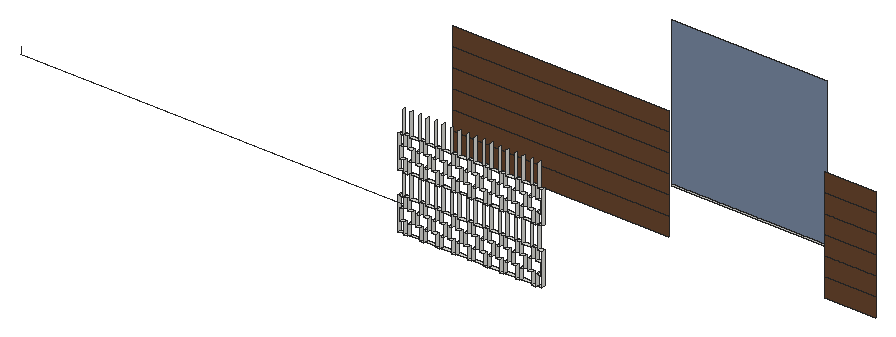
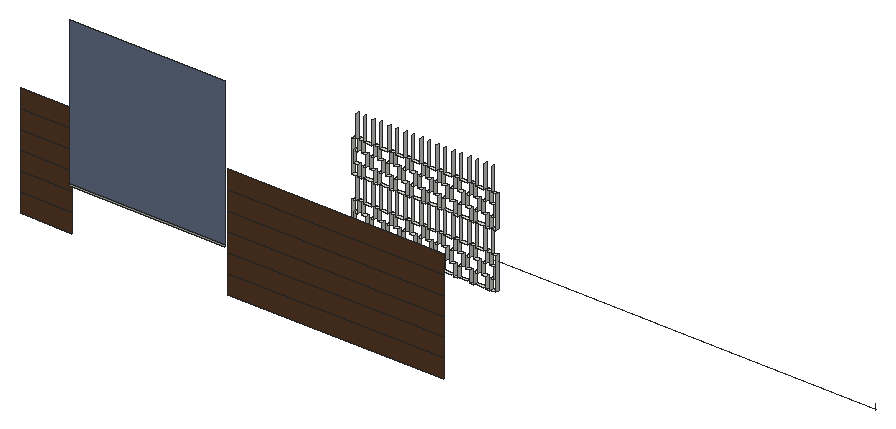
# SketchUp Ruby script. Lengths in inches.
U = 1.inch
M = Sketchup.active_model
def pt(a) = Geom::Point3d.new(a.map { |v| v * U })
def face(e, loops, mat)
  f = e.add_face(loops[0].map { |a| pt(a) })
  loops[1..].each { |l| e.add_face(l.map { |a| pt(a) }).erase! }
  f.material = f.back_material = mat if mat
  f
end
# faces: each face lists its corners as indices into pts; further lists are holes
def faces(e, pts, list, mat = nil) = list.each { |f| face(e, (f[0].is_a?(Array) ? f : [f]).map { |l| l.map { |i| pts[i] } }, mat) }
# xy, xz, yz: faces in a plane at the given z, y or x. An outline is a flat list of corners, or four numbers for a rectangle; further outlines are holes
def ring(l) = l.size == 4 ? [[l[0], l[1]], [l[2], l[1]], [l[2], l[3]], [l[0], l[3]]] : l.each_slice(2).to_a
def flat(e, list, mat, &to3) = list.each { |f| face(e, (f[0].is_a?(Array) ? f : [f]).map { |l| ring(l).map { |u, v| to3.(u, v) } }, mat) }
def xy(e, z, list, mat = nil) = flat(e, list, mat) { |x, y| [x, y, z] }
def xz(e, y, list, mat = nil) = flat(e, list, mat) { |x, z| [x, y, z] }
def yz(e, x, list, mat = nil) = flat(e, list, mat) { |y, z| [x, y, z] }
def lines(e, pts, list) = list.each { |a, b| e.add_line(pt(pts[a]), pt(pts[b])) }
# prism: a flat outline (further loops are holes) pulled along v
def prism(e, loops, v, mat = nil)
  f = face(e, loops, mat); d = Geom::Vector3d.new(v.map { |x| x * U })
  f.pushpull(f.normal.samedirection?(d) ? d.length : -d.length)
end
def box(e, o, s, mat = nil) = prism(e, [[o, [o[0] + s[0], o[1], o[2]], [o[0] + s[0], o[1] + s[1], o[2]], [o[0], o[1] + s[1], o[2]]]], [0, 0, s[2]], mat)
def at(x, y, z, deg = 0) = Geom::Transformation.translation(pt([x, y, z])) * Geom::Transformation.rotation(ORIGIN, Z_AXIS, deg.degrees)
def axes(o, x, y, z) = Geom::Transformation.new([*x, 0, *y, 0, *z, 0, *pt(o).to_a, 1])
def part(name) = M.definitions.add(name)
# library, detail: a bought-in or finely detailed component or shape, given as its bounding box
def library(name, o, s) = part(name).tap { |d| box(d.entities, o, s) }
def detail(e, o, s) = box(e.add_group.entities, o, s)
def put(e, d, t, mat = nil) = e.add_instance(d, t).tap { |i| i.material = mat if mat }
def group(e, t, mat = nil) = e.add_group.tap { |g| g.transformation = t; g.material = mat if mat }.entities
root = M.entities
M.materials.add("Glass_Mirror_01").color = [119, 135, 160]
M.materials.add("Wood_Veneer_15_1K").color = [103, 69, 45]
xy(root,322.72,[[283.14,137.21,284.89,138.74],[290.55,137.21,292.3,138.74],[297.96,137.21,299.71,138.74],[305.37,137.21,307.12,138.74],[312.78,137.21,314.53,138.74],
  [320.1875,137.21,321.94,138.74],[327.6,137.21,329.35,138.74],[335.01,137.21,336.76,138.74],[342.42,137.21,344.17,138.74]])
xy(root,323.12,[[280.31,137.21,282.27,138.74],[285.76,137.21,289.68,138.74],[293.17,137.21,297.09,138.74],[300.58,137.21,304.5,138.74],[307.99,137.21,311.91,138.74],
  [315.4,137.21,319.32,138.74],[322.81,137.21,326.73,138.74],[330.22,137.21,334.14,138.74],[337.63,137.21,341.55,138.74],[345.04,137.21,347,138.74]])
xy(root,327.99,[[281.18,137.21,283.14,138.74],[284.89,137.21,286.85,138.74],[288.59,137.21,290.55,138.74],[292.3,137.21,294.26,138.74],[296,137.21,297.96,138.74],
  [299.71,137.21,301.67,138.74],[303.41,137.21,305.37,138.74],[307.12,137.21,309.08,138.74],[310.82,137.21,312.78,138.74],[314.53,137.21,316.49,138.74],
  [318.23,137.21,320.1875,138.74],[321.94,137.21,323.9,138.74],[325.64,137.21,327.6,138.74],[329.35,137.21,331.31,138.74],[333.05,137.21,335.01,138.74],
  [336.76,137.21,338.72,138.74],[340.46,137.21,342.42,138.74],[344.17,137.21,346.13,138.74]])
xy(root,333.35,[[281.18,137.21,283.14,138.74],[284.89,137.21,286.85,138.74],[288.59,137.21,290.55,138.74],[292.3,137.21,294.26,138.74],[296,137.21,297.96,138.74],
  [299.71,137.21,301.67,138.74],[303.41,137.21,305.37,138.74],[307.12,137.21,309.08,138.74],[310.82,137.21,312.78,138.74],[314.53,137.21,316.49,138.74],
  [318.23,137.21,320.1875,138.74],[321.94,137.21,323.9,138.74],[325.64,137.21,327.6,138.74],[329.35,137.21,331.31,138.74],[333.05,137.21,335.01,138.74],
  [336.76,137.21,338.72,138.74],[340.46,137.21,342.42,138.74],[344.17,137.21,346.13,138.74]])
xy(root,338.22,[[280.31,137.21,282.27,138.74],[285.76,137.21,289.68,138.74],[293.17,137.21,297.09,138.74],[300.58,137.21,304.5,138.74],[307.99,137.21,311.91,138.74],
  [315.4,137.21,319.32,138.74],[322.81,137.21,326.73,138.74],[330.22,137.21,334.14,138.74],[337.63,137.21,341.55,138.74],[345.04,137.21,347,138.74]])
xy(root,338.62,[[283.14,137.21,284.89,138.74],[290.55,137.21,292.3,138.74],[297.96,137.21,299.71,138.74],[305.37,137.21,307.12,138.74],[312.78,137.21,314.53,138.74],
  [320.1875,137.21,321.94,138.74],[327.6,137.21,329.35,138.74],[335.01,137.21,336.76,138.74],[342.42,137.21,344.17,138.74]])
xy(root,348.35,[[283.14,137.21,284.89,138.74],[290.55,137.21,292.3,138.74],[297.96,137.21,299.71,138.74],[305.37,137.21,307.12,138.74],[312.78,137.21,314.53,138.74],
  [320.1875,137.21,321.94,138.74],[327.6,137.21,329.35,138.74],[335.01,137.21,336.76,138.74],[342.42,137.21,344.17,138.74]])
xy(root,348.75,[[280.31,137.21,282.27,138.74],[285.76,137.21,289.68,138.74],[293.17,137.21,297.09,138.74],[300.58,137.21,304.5,138.74],[307.99,137.21,311.91,138.74],
  [315.4,137.21,319.32,138.74],[322.81,137.21,326.73,138.74],[330.22,137.21,334.14,138.74],[337.63,137.21,341.55,138.74],[345.04,137.21,347,138.74]])
xy(root,353.62,[[281.18,137.21,283.14,138.74],[284.89,137.21,286.85,138.74],[288.59,137.21,290.55,138.74],[292.3,137.21,294.26,138.74],[296,137.21,297.96,138.74],
  [299.71,137.21,301.67,138.74],[303.41,137.21,305.37,138.74],[307.12,137.21,309.08,138.74],[310.82,137.21,312.78,138.74],[314.53,137.21,316.49,138.74],
  [318.23,137.21,320.1875,138.74],[321.94,137.21,323.9,138.74],[325.64,137.21,327.6,138.74],[329.35,137.21,331.31,138.74],[333.05,137.21,335.01,138.74],
  [336.76,137.21,338.72,138.74],[340.46,137.21,342.42,138.74],[344.17,137.21,346.13,138.74]])
xy(root,358.98,[[281.18,137.21,283.14,138.74],[284.89,137.21,286.85,138.74],[288.59,137.21,290.55,138.74],[292.3,137.21,294.26,138.74],[296,137.21,297.96,138.74],
  [299.71,137.21,301.67,138.74],[303.41,137.21,305.37,138.74],[307.12,137.21,309.08,138.74],[310.82,137.21,312.78,138.74],[314.53,137.21,316.49,138.74],
  [318.23,137.21,320.1875,138.74],[321.94,137.21,323.9,138.74],[325.64,137.21,327.6,138.74],[329.35,137.21,331.31,138.74],[333.05,137.21,335.01,138.74],
  [336.76,137.21,338.72,138.74],[340.46,137.21,342.42,138.74],[344.17,137.21,346.13,138.74]])
xy(root,363.84,[[280.31,137.21,282.27,138.74],[285.76,137.21,289.68,138.74],[293.17,137.21,297.09,138.74],[300.58,137.21,304.5,138.74],[307.99,137.21,311.91,138.74],
  [315.4,137.21,319.32,138.74],[322.81,137.21,326.73,138.74],[330.22,137.21,334.14,138.74],[337.63,137.21,341.55,138.74],[345.04,137.21,347,138.74]])
xy(root,364.24,[[283.14,137.21,284.89,138.74],[290.55,137.21,292.3,138.74],[297.96,137.21,299.71,138.74],[305.37,137.21,307.12,138.74],[312.78,137.21,314.53,138.74],
  [320.1875,137.21,321.94,138.74],[327.6,137.21,329.35,138.74],[335.01,137.21,336.76,138.74],[342.42,137.21,344.17,138.74]])
xz(root,198,[[256.9,321.28,357,329.96],[429,321.28,453,329.96],[256.9,329.96,357,338.64],[429,329.96,453,338.64],[256.9,338.64,357,347.32],
  [429,338.64,453,347.32],[256.9,347.32,357,356],[429,347.32,453,356],[256.9,356,357,364.68],[429,356,453,364.68],
  [256.9,364.68,357,373.36],[429,364.68,453,373.36]],"Wood_Veneer_15_1K")
xz(root,199.5,[[357,341.52,429,342.52]])
xz(root,199.5,[[357,342.52,429,410.35]],"Glass_Mirror_01")
yz(root,280.31,[[137.21,323.12,138.74,338.22],[137.21,348.75,138.74,363.84]])
yz(root,281.18,[[137.21,327.99,138.74,333.35],[137.21,353.62,138.74,358.98]])
yz(root,282.27,[[137.21,338.22,138.74,348.75],[137.21,363.84,138.74,374.38]])
yz(root,283.14,[[137.21,322.72,138.74,327.99],[137.21,333.35,138.74,338.62],[137.21,348.35,138.74,353.62],[137.21,358.98,138.74,364.24]])
yz(root,284.89,[[137.21,322.72,138.74,327.99],[137.21,333.35,138.74,338.62],[137.21,348.35,138.74,353.62],[137.21,358.98,138.74,364.24]])
yz(root,285.76,[[137.21,338.22,138.74,348.75],[137.21,363.84,138.74,374.38]])
yz(root,286.85,[[137.21,327.99,138.74,333.35],[137.21,353.62,138.74,358.98]])
yz(root,288.59,[[137.21,327.99,138.74,333.35],[137.21,353.62,138.74,358.98]])
yz(root,289.68,[[137.21,338.22,138.74,348.75],[137.21,363.84,138.74,374.38]])
yz(root,290.55,[[137.21,322.72,138.74,327.99],[137.21,333.35,138.74,338.62],[137.21,348.35,138.74,353.62],[137.21,358.98,138.74,364.24]])
yz(root,292.3,[[137.21,322.72,138.74,327.99],[137.21,333.35,138.74,338.62],[137.21,348.35,138.74,353.62],[137.21,358.98,138.74,364.24]])
yz(root,293.17,[[137.21,338.22,138.74,348.75],[137.21,363.84,138.74,374.38]])
yz(root,294.26,[[137.21,327.99,138.74,333.35],[137.21,353.62,138.74,358.98]])
yz(root,296,[[137.21,327.99,138.74,333.35],[137.21,353.62,138.74,358.98]])
yz(root,297.09,[[137.21,338.22,138.74,348.75],[137.21,363.84,138.74,374.38]])
yz(root,297.96,[[137.21,322.72,138.74,327.99],[137.21,333.35,138.74,338.62],[137.21,348.35,138.74,353.62],[137.21,358.98,138.74,364.24]])
yz(root,299.71,[[137.21,322.72,138.74,327.99],[137.21,333.35,138.74,338.62],[137.21,348.35,138.74,353.62],[137.21,358.98,138.74,364.24]])
yz(root,300.58,[[137.21,338.22,138.74,348.75],[137.21,363.84,138.74,374.38]])
yz(root,301.67,[[137.21,327.99,138.74,333.35],[137.21,353.62,138.74,358.98]])
yz(root,303.41,[[137.21,327.99,138.74,333.35],[137.21,353.62,138.74,358.98]])
yz(root,304.5,[[137.21,338.22,138.74,348.75],[137.21,363.84,138.74,374.38]])
yz(root,305.37,[[137.21,322.72,138.74,327.99],[137.21,333.35,138.74,338.62],[137.21,348.35,138.74,353.62],[137.21,358.98,138.74,364.24]])
yz(root,307.12,[[137.21,322.72,138.74,327.99],[137.21,333.35,138.74,338.62],[137.21,348.35,138.74,353.62],[137.21,358.98,138.74,364.24]])
yz(root,307.99,[[137.21,338.22,138.74,348.75],[137.21,363.84,138.74,374.38]])
yz(root,309.08,[[137.21,327.99,138.74,333.35],[137.21,353.62,138.74,358.98]])
yz(root,310.82,[[137.21,327.99,138.74,333.35],[137.21,353.62,138.74,358.98]])
yz(root,311.91,[[137.21,338.22,138.74,348.75],[137.21,363.84,138.74,374.38]])
yz(root,312.78,[[137.21,322.72,138.74,327.99],[137.21,333.35,138.74,338.62],[137.21,348.35,138.74,353.62],[137.21,358.98,138.74,364.24]])
yz(root,314.53,[[137.21,322.72,138.74,327.99],[137.21,333.35,138.74,338.62],[137.21,348.35,138.74,353.62],[137.21,358.98,138.74,364.24]])
yz(root,315.4,[[137.21,338.22,138.74,348.75],[137.21,363.84,138.74,374.38]])
yz(root,316.49,[[137.21,327.99,138.74,333.35],[137.21,353.62,138.74,358.98]])
yz(root,318.23,[[137.21,327.99,138.74,333.35],[137.21,353.62,138.74,358.98]])
yz(root,319.32,[[137.21,338.22,138.74,348.75],[137.21,363.84,138.74,374.38]])
yz(root,320.1875,[[137.21,322.72,138.74,327.99],[137.21,333.35,138.74,338.62],[137.21,348.35,138.74,353.62],[137.21,358.98,138.74,364.24]])
yz(root,321.94,[[137.21,322.72,138.74,327.99],[137.21,333.35,138.74,338.62],[137.21,348.35,138.74,353.62],[137.21,358.98,138.74,364.24]])
yz(root,322.81,[[137.21,338.22,138.74,348.75],[137.21,363.84,138.74,374.38]])
yz(root,323.9,[[137.21,327.99,138.74,333.35],[137.21,353.62,138.74,358.98]])
yz(root,325.64,[[137.21,327.99,138.74,333.35],[137.21,353.62,138.74,358.98]])
yz(root,326.73,[[137.21,338.22,138.74,348.75],[137.21,363.84,138.74,374.38]])
yz(root,327.6,[[137.21,322.72,138.74,327.99],[137.21,333.35,138.74,338.62],[137.21,348.35,138.74,353.62],[137.21,358.98,138.74,364.24]])
yz(root,329.35,[[137.21,322.72,138.74,327.99],[137.21,333.35,138.74,338.62],[137.21,348.35,138.74,353.62],[137.21,358.98,138.74,364.24]])
yz(root,330.22,[[137.21,338.22,138.74,348.75],[137.21,363.84,138.74,374.38]])
yz(root,331.31,[[137.21,327.99,138.74,333.35],[137.21,353.62,138.74,358.98]])
yz(root,333.05,[[137.21,327.99,138.74,333.35],[137.21,353.62,138.74,358.98]])
yz(root,334.14,[[137.21,338.22,138.74,348.75],[137.21,363.84,138.74,374.38]])
yz(root,335.01,[[137.21,322.72,138.74,327.99],[137.21,333.35,138.74,338.62],[137.21,348.35,138.74,353.62],[137.21,358.98,138.74,364.24]])
yz(root,336.76,[[137.21,322.72,138.74,327.99],[137.21,333.35,138.74,338.62],[137.21,348.35,138.74,353.62],[137.21,358.98,138.74,364.24]])
yz(root,337.63,[[137.21,338.22,138.74,348.75],[137.21,363.84,138.74,374.38]])
yz(root,338.72,[[137.21,327.99,138.74,333.35],[137.21,353.62,138.74,358.98]])
yz(root,340.46,[[137.21,327.99,138.74,333.35],[137.21,353.62,138.74,358.98]])
yz(root,341.55,[[137.21,338.22,138.74,348.75],[137.21,363.84,138.74,374.38]])
yz(root,342.42,[[137.21,322.72,138.74,327.99],[137.21,333.35,138.74,338.62],[137.21,348.35,138.74,353.62],[137.21,358.98,138.74,364.24]])
yz(root,344.17,[[137.21,322.72,138.74,327.99],[137.21,333.35,138.74,338.62],[137.21,348.35,138.74,353.62],[137.21,358.98,138.74,364.24]])
yz(root,345.04,[[137.21,338.22,138.74,348.75],[137.21,363.84,138.74,374.38]])
yz(root,346.13,[[137.21,327.99,138.74,333.35],[137.21,353.62,138.74,358.98]])
yz(root,347,[[137.21,323.12,138.74,338.22],[137.21,348.75,138.74,363.84]])
p = [[105.48,137.9375,335.1],[105.48,137.9375,338],[105.48,137.1875,335.2],[282.125,137.21,335.2]]
lines(root,p,[[0,1],[2,3]])
